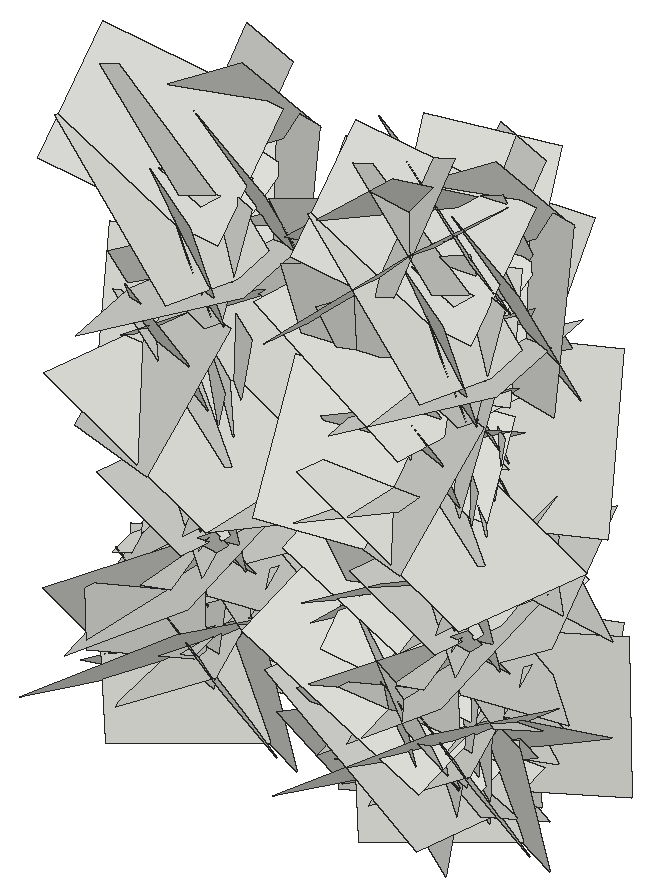
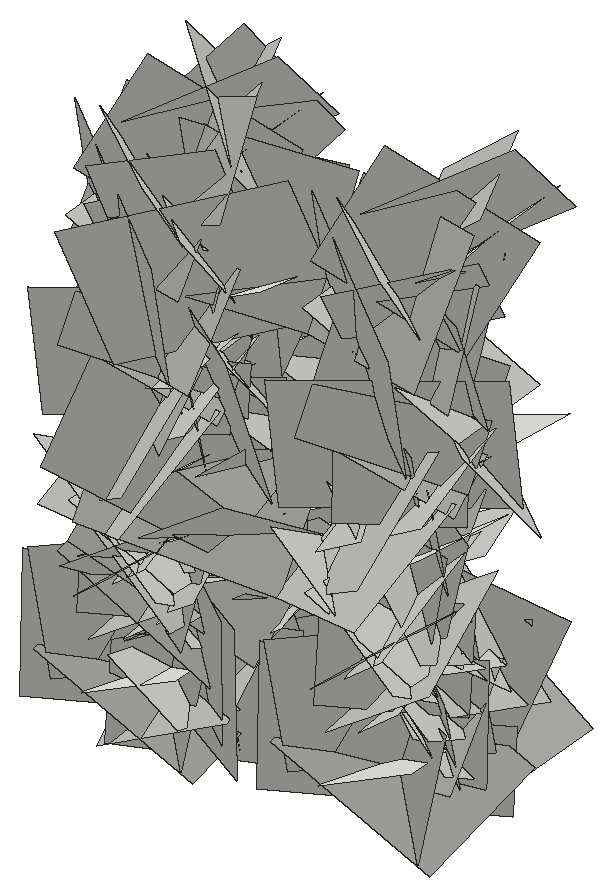
# SketchUp Ruby script. Lengths in inches.
U = 1.inch
M = Sketchup.active_model
def pt(a) = Geom::Point3d.new(a.map { |v| v * U })
def face(e, loops, mat)
  f = e.add_face(loops[0].map { |a| pt(a) })
  loops[1..].each { |l| e.add_face(l.map { |a| pt(a) }).erase! }
  f.material = f.back_material = mat if mat
  f
end
# faces: each face lists its corners as indices into pts; further lists are holes
def faces(e, pts, list, mat = nil) = list.each { |f| face(e, (f[0].is_a?(Array) ? f : [f]).map { |l| l.map { |i| pts[i] } }, mat) }
# xy, xz, yz: faces in a plane at the given z, y or x. An outline is a flat list of corners, or four numbers for a rectangle; further outlines are holes
def ring(l) = l.size == 4 ? [[l[0], l[1]], [l[2], l[1]], [l[2], l[3]], [l[0], l[3]]] : l.each_slice(2).to_a
def flat(e, list, mat, &to3) = list.each { |f| face(e, (f[0].is_a?(Array) ? f : [f]).map { |l| ring(l).map { |u, v| to3.(u, v) } }, mat) }
def xy(e, z, list, mat = nil) = flat(e, list, mat) { |x, y| [x, y, z] }
def xz(e, y, list, mat = nil) = flat(e, list, mat) { |x, z| [x, y, z] }
def yz(e, x, list, mat = nil) = flat(e, list, mat) { |y, z| [x, y, z] }
def lines(e, pts, list) = list.each { |a, b| e.add_line(pt(pts[a]), pt(pts[b])) }
# prism: a flat outline (further loops are holes) pulled along v
def prism(e, loops, v, mat = nil)
  f = face(e, loops, mat); d = Geom::Vector3d.new(v.map { |x| x * U })
  f.pushpull(f.normal.samedirection?(d) ? d.length : -d.length)
end
def box(e, o, s, mat = nil) = prism(e, [[o, [o[0] + s[0], o[1], o[2]], [o[0] + s[0], o[1] + s[1], o[2]], [o[0], o[1] + s[1], o[2]]]], [0, 0, s[2]], mat)
def at(x, y, z, deg = 0) = Geom::Transformation.translation(pt([x, y, z])) * Geom::Transformation.rotation(ORIGIN, Z_AXIS, deg.degrees)
def axes(o, x, y, z) = Geom::Transformation.new([*x, 0, *y, 0, *z, 0, *pt(o).to_a, 1])
def part(name) = M.definitions.add(name)
# library, detail: a bought-in or finely detailed component or shape, given as its bounding box
def library(name, o, s) = part(name).tap { |d| box(d.entities, o, s) }
def detail(e, o, s) = box(e.add_group.entities, o, s)
def put(e, d, t, mat = nil) = e.add_instance(d, t).tap { |i| i.material = mat if mat }
def group(e, t, mat = nil) = e.add_group.tap { |g| g.transformation = t; g.material = mat if mat }.entities
root = M.entities
c1 = part("Component\#6")
p = [[0.01,0,0],[0,3.24,4.54],[4.32,3.24,4.54],[4.33,0,0]]
faces(c1.entities,p,[[0,1,2,3]])
put(root,c1,axes([414.68,169.73,5.36],[-0.07377,0.11031,-0.61615],[-0.06228,-0.61836,-0.10407],[-0.66058,0.04598,0.07863]))
put(root,c1,axes([420.52,169.73,5.36],[0.07377,0.11031,-0.61615],[0.06228,-0.61836,-0.10407],[0.66058,0.04598,0.07863]))
put(root,c1,axes([424.49,169.73,5.36],[-0.07377,0.11031,-0.61615],[-0.06228,-0.61836,-0.10407],[-0.66058,0.04598,0.07863]))
put(root,c1,axes([414.68,170.45,6.95],[0.13562,-0.59571,0.16409],[-0.06684,0.15411,0.60864],[-0.65155,-0.13981,-0.02828]))
put(root,c1,axes([420.52,170.45,6.95],[-0.13562,-0.59571,0.16409],[0.06684,0.15411,0.60864],[0.65155,-0.13981,-0.02828]))
put(root,c1,axes([424.49,170.45,6.95],[0.13562,-0.59571,0.16409],[-0.06684,0.15411,0.60864],[-0.65155,-0.13981,-0.02828]))
put(root,c1,axes([410.71,172.51,13.7],[-0.18405,-0.71312,-0.93832],[-0.0125,-0.94735,0.72216],[1.2492,-0.11455,-0.13102]))
put(root,c1,axes([424.49,172.51,13.7],[0.18405,-0.71312,-0.93832],[0.0125,-0.94735,0.72216],[-1.2492,-0.11455,-0.13102]))
put(root,c1,axes([420.52,172.51,13.7],[-0.18405,-0.71312,-0.93832],[-0.0125,-0.94735,0.72216],[1.2492,-0.11455,-0.13102]))
put(root,c1,axes([410.71,166.89,12.83],[0.13197,1.26874,-0.04114],[0.28106,-0.06642,-1.24587],[1.31589,-0.11305,0.27023]))
put(root,c1,axes([424.49,166.89,12.83],[-0.13197,1.26874,-0.04114],[-0.28106,-0.06642,-1.24587],[-1.31589,-0.11305,0.27023]))
put(root,c1,axes([420.52,166.89,12.83],[0.13197,1.26874,-0.04114],[0.28106,-0.06642,-1.24587],[1.31589,-0.11305,0.27023]))
put(root,c1,axes([414.68,170.4375,18.81],[0.19883,-0.70321,0.38228],[0.06935,0.40479,0.71252],[-0.84558,-0.13215,0.14832]))
put(root,c1,axes([420.52,170.4375,18.81],[-0.19883,-0.70321,0.38228],[-0.06935,0.40479,0.71252],[0.84558,-0.13215,0.14832]))
put(root,c1,axes([424.49,170.4375,18.81],[0.19883,-0.70321,0.38228],[0.06935,0.40479,0.71252],[-0.84558,-0.13215,0.14832]))
put(root,c1,axes([410.71,172.01,0.23],[-0.18306,-1.21621,0.26629],[-0.00588,0.26959,1.22768],[1.31971,-0.16751,0.04241]))
put(root,c1,axes([424.49,172.01,0.23],[0.18306,-1.21621,0.26629],[0.00588,0.26959,1.22768],[-1.31971,-0.16751,0.04241]))
put(root,c1,axes([420.52,172.01,0.23],[-0.18306,-1.21621,0.26629],[-0.00588,0.26959,1.22768],[1.31971,-0.16751,0.04241]))
put(root,c1,axes([410.71,167.43,21.54],[0.05686,1.16606,-0.16138],[-0.18622,-0.15181,-1.15529],[1.23383,-0.07665,-0.16693]))
put(root,c1,axes([424.49,167.43,21.54],[-0.05686,1.16606,-0.16138],[0.18622,-0.15181,-1.15529],[-1.23383,-0.07665,-0.16693]))
put(root,c1,axes([420.52,167.43,21.54],[0.05686,1.16606,-0.16138],[-0.18622,-0.15181,-1.15529],[1.23383,-0.07665,-0.16693]))
put(root,c1,axes([410.71,170.29,20.28],[0.01759,0.35165,-0.94572],[0.09141,-0.94289,-0.34909],[1.06561,0.07508,0.04555]))
put(root,c1,axes([424.49,170.29,20.28],[-0.01759,0.35165,-0.94572],[-0.09141,-0.94289,-0.34909],[-1.06561,0.07508,0.04555]))
put(root,c1,axes([420.52,170.29,20.28],[0.01759,0.35165,-0.94572],[0.09141,-0.94289,-0.34909],[1.06561,0.07508,0.04555]))
put(root,c1,axes([410.71,166.61,20.4],[0.01588,0.7114,0.79833],[-0.18087,0.78977,-0.70057],[1.11894,0.11757,-0.12458]))
put(root,c1,axes([424.49,166.61,20.4],[-0.01588,0.7114,0.79833],[0.18087,0.78977,-0.70057],[-1.11894,0.11757,-0.12458]))
put(root,c1,axes([420.52,166.61,20.4],[0.01588,0.7114,0.79833],[-0.18087,0.78977,-0.70057],[1.11894,0.11757,-0.12458]))
put(root,c1,axes([414.68,169.875,11.58],[0.08121,-0.31714,0.54408],[-0.11401,0.53345,0.32609],[-0.65774,-0.13162,0.01065]))
put(root,c1,axes([420.52,169.875,11.58],[-0.08121,-0.31714,0.54408],[0.11401,0.53345,0.32609],[0.65774,-0.13162,0.01065]))
put(root,c1,axes([424.49,169.875,11.58],[0.08121,-0.31714,0.54408],[-0.11401,0.53345,0.32609],[-0.65774,-0.13162,0.01065]))
put(root,c1,axes([410.71,169.82,1.95],[-0.02915,-0.64251,0.76006],[-0.08177,0.75943,0.6392],[1.05178,0.04123,0.07076]))
put(root,c1,axes([424.49,169.82,1.95],[0.02915,-0.64251,0.76006],[0.08177,0.75943,0.6392],[-1.05178,0.04123,0.07076]))
put(root,c1,axes([420.52,169.82,1.95],[-0.02915,-0.64251,0.76006],[-0.08177,0.75943,0.6392],[1.05178,0.04123,0.07076]))
put(root,c1,axes([410.71,173.1,4.27],[0.006,-1.20261,-0.38975],[-0.07836,-0.3894,1.20046],[1.33775,-0.01742,0.07206]))
put(root,c1,axes([424.49,173.1,4.27],[-0.006,-1.20261,-0.38975],[0.07836,-0.3894,1.20046],[-1.33775,-0.01742,0.07206]))
put(root,c1,axes([420.52,173.1,4.27],[0.006,-1.20261,-0.38975],[-0.07836,-0.3894,1.20046],[1.33775,-0.01742,0.07206]))
put(root,c1,axes([414.68,169.57,7.53],[-0.02893,-0.34038,0.60393],[0.06424,0.60091,0.34142],[-0.73203,0.06619,0.00609]))
put(root,c1,axes([420.52,169.57,7.53],[0.02893,-0.34038,0.60393],[-0.06424,0.60091,0.34142],[0.73203,0.06619,0.00609]))
put(root,c1,axes([424.49,169.57,7.53],[-0.02893,-0.34038,0.60393],[0.06424,0.60091,0.34142],[-0.73203,0.06619,0.00609]))
put(root,c1,axes([410.71,172.68,14.25],[0.15371,-1.16437,-0.05617],[0.14183,-0.0396,1.1664],[1.22751,0.15038,-0.12774]))
put(root,c1,axes([424.49,172.68,14.25],[-0.15371,-1.16437,-0.05617],[-0.14183,-0.0396,1.1664],[-1.22751,0.15038,-0.12774]))
put(root,c1,axes([420.52,172.68,14.25],[0.15371,-1.16437,-0.05617],[0.14183,-0.0396,1.1664],[1.22751,0.15038,-0.12774]))
put(root,c1,axes([414.68,172.08,18.68],[0.05145,-0.65016,0.07549],[-0.09383,0.06848,0.64671],[-0.68743,-0.05801,-0.08262]))
put(root,c1,axes([424.49,172.08,18.68],[0.05145,-0.65016,0.07549],[-0.09383,0.06848,0.64671],[-0.68743,-0.05801,-0.08262]))
put(root,c1,axes([420.52,172.08,18.68],[-0.05145,-0.65016,0.07549],[0.09383,0.06848,0.64671],[0.68743,-0.05801,-0.08262]))
put(root,c1,axes([414.68,168.08,6.15],[0.10311,0.69666,0.5447],[0.01855,0.54636,-0.70191],[-0.9372,0.08746,0.04604]))
put(root,c1,axes([420.52,168.08,6.15],[-0.10311,0.69666,0.5447],[-0.01855,0.54636,-0.70191],[0.9372,0.08746,0.04604]))
put(root,c1,axes([424.49,168.08,6.15],[0.10311,0.69666,0.5447],[0.01855,0.54636,-0.70191],[-0.9372,0.08746,0.04604]))
put(root,c1,axes([410.71,170.37,5.28],[-0.04044,0.69271,-0.86885],[0.14808,-0.85947,-0.69137],[1.16852,0.13289,0.05755]))
put(root,c1,axes([424.49,170.37,5.28],[0.04044,0.69271,-0.86885],[-0.14808,-0.85947,-0.69137],[-1.16852,0.13289,0.05755]))
put(root,c1,axes([420.52,170.37,5.28],[-0.04044,0.69271,-0.86885],[0.14808,-0.85947,-0.69137],[1.16852,0.13289,0.05755]))
put(root,c1,axes([410.71,171.61,19.65],[-0.05512,0.44879,-0.89687],[-0.12411,-0.89465,-0.44089],[1.05579,-0.08174,-0.09865]))
put(root,c1,axes([424.49,171.61,19.65],[0.05512,0.44879,-0.89687],[0.12411,-0.89465,-0.44089],[-1.05579,-0.08174,-0.09865]))
put(root,c1,axes([420.52,171.61,19.65],[-0.05512,0.44879,-0.89687],[-0.12411,-0.89465,-0.44089],[1.05579,-0.08174,-0.09865]))
put(root,c1,axes([410.71,172.8125,18.6875],[-0.10377,-0.25363,-0.96814],[0.17625,-0.96337,0.23557],[1.04612,0.13715,-0.13572]))
put(root,c1,axes([424.49,172.8125,18.6875],[0.10377,-0.25363,-0.96814],[-0.17625,-0.96337,0.23557],[-1.04612,0.13715,-0.13572]))
put(root,c1,axes([420.52,172.8125,18.6875],[-0.10377,-0.25363,-0.96814],[0.17625,-0.96337,0.23557],[1.04612,0.13715,-0.13572]))
put(root,c1,axes([410.71,173.43,2.26],[0.13173,-0.86629,-0.47025],[-0.00519,-0.47451,0.87284],[1.04483,0.10686,0.06363]))
put(root,c1,axes([424.49,173.43,2.26],[-0.13173,-0.86629,-0.47025],[0.00519,-0.47451,0.87284],[-1.04483,0.10686,0.06363]))
put(root,c1,axes([420.52,173.43,2.26],[0.13173,-0.86629,-0.47025],[-0.00519,-0.47451,0.87284],[1.04483,0.10686,0.06363]))
put(root,c1,axes([414.68,172.62,2.82],[0.11022,-0.07985,-0.84847],[-0.01268,-0.85481,0.07898],[-0.90326,0.00226,-0.10464]))
put(root,c1,axes([420.52,172.62,2.82],[-0.11022,-0.07985,-0.84847],[0.01268,-0.85481,0.07898],[0.90326,0.00226,-0.10464]))
put(root,c1,axes([424.49,172.62,2.82],[0.11022,-0.07985,-0.84847],[-0.01268,-0.85481,0.07898],[-0.90326,0.00226,-0.10464]))
put(root,c1,axes([424.49,172.18,10.26],[-0.13568,0.14362,-0.9313],[-0.0793,-0.93844,-0.13444],[-0.9957,0.05517,0.13761]))
put(root,c1,axes([410.71,172.18,10.26],[0.13568,0.14362,-0.9313],[0.0793,-0.93844,-0.13444],[0.9957,0.05517,0.13761]))
put(root,c1,axes([420.52,172.18,10.26],[0.13568,0.14362,-0.9313],[0.0793,-0.93844,-0.13444],[0.9957,0.05517,0.13761]))
put(root,c1,axes([414.68,169.25,3.37],[0.12984,0.58451,0.34416],[0.01188,0.34794,-0.59491],[-0.71891,0.11132,0.05233]))
put(root,c1,axes([420.52,169.25,3.37],[-0.12984,0.58451,0.34416],[-0.01188,0.34794,-0.59491],[0.71891,0.11132,0.05233]))
put(root,c1,axes([424.49,169.25,3.37],[0.12984,0.58451,0.34416],[0.01188,0.34794,-0.59491],[-0.71891,0.11132,0.05233]))
put(root,c1,axes([410.71,174.625,6.88],[0.07025,-1.10898,-0.49527],[-0.16839,-0.49966,1.09755],[1.27636,-0.00489,0.17206]))
put(root,c1,axes([424.49,174.625,6.88],[-0.07025,-1.10898,-0.49527],[0.16839,-0.49966,1.09755],[-1.27636,-0.00489,0.17206]))
put(root,c1,axes([420.52,174.625,6.88],[0.07025,-1.10898,-0.49527],[-0.16839,-0.49966,1.09755],[1.27636,-0.00489,0.17206]))
put(root,c1,axes([410.71,173.47,4.9],[0.07332,-0.2848,-0.87141],[-0.0336,-0.87411,0.28317],[0.9712,-0.00874,0.07558]))
put(root,c1,axes([424.49,173.47,4.9],[-0.07332,-0.2848,-0.87141],[0.0336,-0.87411,0.28317],[-0.9712,-0.00874,0.07558]))
put(root,c1,axes([420.52,173.47,4.9],[0.07332,-0.2848,-0.87141],[-0.0336,-0.87411,0.28317],[0.9712,-0.00874,0.07558]))
put(root,c1,axes([414.68,169.67,8.54],[0.12628,0.08221,0.86907],[0.11161,0.86937,-0.09667],[-0.91857,0.11693,0.10773]))
put(root,c1,axes([420.52,169.67,8.54],[-0.12628,0.08221,0.86907],[-0.11161,0.86937,-0.09667],[0.91857,0.11693,0.10773]))
put(root,c1,axes([424.49,169.67,8.54],[0.12628,0.08221,0.86907],[0.11161,0.86937,-0.09667],[-0.91857,0.11693,0.10773]))
put(root,c1,axes([414.68,173.61,18.42],[-0.00387,-0.64214,-0.38262],[-0.01033,-0.38255,0.64212],[-0.79227,0.00812,-0.0065]))
put(root,c1,axes([420.52,173.61,18.42],[0.00387,-0.64214,-0.38262],[0.01033,-0.38255,0.64212],[0.79227,0.00812,-0.0065]))
put(root,c1,axes([424.49,173.61,18.42],[-0.00387,-0.64214,-0.38262],[-0.01033,-0.38255,0.64212],[-0.79227,0.00812,-0.0065]))
put(root,c1,axes([410.71,173.47,6.03],[-0.02519,-0.71274,-0.22366],[0.1783,-0.22314,0.69319],[0.7715,0.02829,-0.1675]))
put(root,c1,axes([424.49,173.47,6.03],[0.02519,-0.71274,-0.22366],[-0.1783,-0.22314,0.69319],[-0.7715,0.02829,-0.1675]))
put(root,c1,axes([420.52,173.47,6.03],[-0.02519,-0.71274,-0.22366],[0.1783,-0.22314,0.69319],[0.7715,0.02829,-0.1675]))
put(root,c1,axes([410.71,170.23,14.27],[-0.02775,1.05616,-0.50439],[-0.01222,-0.50473,-1.05626],[1.24058,0.01865,-0.02169]))
put(root,c1,axes([424.49,170.23,14.27],[0.02775,1.05616,-0.50439],[0.01222,-0.50473,-1.05626],[-1.24058,0.01865,-0.02169]))
put(root,c1,axes([420.52,170.23,14.27],[-0.02775,1.05616,-0.50439],[-0.01222,-0.50473,-1.05626],[1.24058,0.01865,-0.02169]))
put(root,c1,axes([410.71,172.3,17.31],[-0.17712,-0.66279,0.75583],[0.05377,0.75967,0.67737],[1.06423,-0.14869,0.09157]))
put(root,c1,axes([424.49,172.3,17.31],[0.17712,-0.66279,0.75583],[-0.05377,0.75967,0.67737],[-1.06423,-0.14869,0.09157]))
put(root,c1,axes([420.52,172.3,17.31],[-0.17712,-0.66279,0.75583],[0.05377,0.75967,0.67737],[1.06423,-0.14869,0.09157]))
put(root,c1,axes([410.71,171.9,21.66],[0.05821,0.63814,-1.10333],[0.23209,-1.09266,-0.62107],[1.33097,0.16262,0.15656]))
put(root,c1,axes([424.49,171.9,21.66],[-0.05821,0.63814,-1.10333],[-0.23209,-1.09266,-0.62107],[-1.33097,0.16262,0.15656]))
put(root,c1,axes([420.52,171.9,21.66],[0.05821,0.63814,-1.10333],[0.23209,-1.09266,-0.62107],[1.33097,0.16262,0.15656]))
put(root,c1,axes([414.68,171.64,6.09],[0.04085,-0.22846,0.61977],[-0.06336,0.61707,0.23119],[-0.6973,-0.06945,0.0153]))
put(root,c1,axes([420.52,171.64,6.09],[-0.04085,-0.22846,0.61977],[0.06336,0.61707,0.23119],[0.6973,-0.06945,0.0153]))
put(root,c1,axes([424.49,171.64,6.09],[0.04085,-0.22846,0.61977],[-0.06336,0.61707,0.23119],[-0.6973,-0.06945,0.0153]))
put(root,c1,axes([410.71,170.14,10.52],[0.06349,0.95893,0.01002],[-0.03302,0.01198,-0.96028],[1.01599,-0.05954,-0.03183]))
put(root,c1,axes([424.49,170.14,10.52],[-0.06349,0.95893,0.01002],[0.03302,0.01198,-0.96028],[-1.01599,-0.05954,-0.03183]))
put(root,c1,axes([420.52,170.14,10.52],[0.06349,0.95893,0.01002],[-0.03302,0.01198,-0.96028],[1.01599,-0.05954,-0.03183]))
put(root,c1,axes([414.68,174.87,19.3],[0.1513,-0.51657,-0.73784],[0.06675,-0.7395,0.52991],[-0.9524,-0.13389,-0.08008]))
put(root,c1,axes([420.52,174.87,19.3],[-0.1513,-0.51657,-0.73784],[-0.06675,-0.7395,0.52991],[0.9524,-0.13389,-0.08008]))
put(root,c1,axes([424.49,174.87,19.3],[0.1513,-0.51657,-0.73784],[0.06675,-0.7395,0.52991],[-0.9524,-0.13389,-0.08008]))
put(root,c1,axes([410.71,172.92,11.6],[0.15777,-0.72106,0.34948],[-0.01112,0.35368,0.73418],[0.84929,0.13857,-0.05531]))
put(root,c1,axes([424.49,172.92,11.6],[-0.15777,-0.72106,0.34948],[0.01112,0.35368,0.73418],[-0.84929,0.13857,-0.05531]))
put(root,c1,axes([420.52,172.92,11.6],[0.15777,-0.72106,0.34948],[-0.01112,0.35368,0.73418],[0.84929,0.13857,-0.05531]))
put(root,c1,axes([410.71,169.35,10.4],[-0.15861,0.37048,1.309],[0.06067,1.31744,-0.36632],[1.44077,-0.01469,0.15953]))
put(root,c1,axes([424.49,169.35,10.4],[0.15861,0.37048,1.309],[-0.06067,1.31744,-0.36632],[-1.44077,-0.01469,0.15953]))
put(root,c1,axes([420.52,169.35,10.4],[-0.15861,0.37048,1.309],[0.06067,1.31744,-0.36632],[1.44077,-0.01469,0.15953]))
put(root,c1,axes([410.71,171.5,10.51],[0.09816,1.08592,-0.68794],[-0.27584,-0.65961,-1.07622],[1.33441,-0.21623,-0.17187]))
put(root,c1,axes([424.49,171.5,10.51],[-0.09816,1.08592,-0.68794],[0.27584,-0.65961,-1.07622],[-1.33441,-0.21623,-0.17187]))
put(root,c1,axes([420.52,171.5,10.51],[0.09816,1.08592,-0.68794],[-0.27584,-0.65961,-1.07622],[1.33441,-0.21623,-0.17187]))
put(root,c1,axes([410.71,170.67,8.7],[-0.18467,1.04701,-0.56036],[-0.0341,-0.57031,-1.0556],[1.25832,0.1382,-0.11085]))
put(root,c1,axes([424.49,170.67,8.7],[0.18467,1.04701,-0.56036],[0.0341,-0.57031,-1.0556],[-1.25832,0.1382,-0.11085]))
put(root,c1,axes([420.52,170.67,8.7],[-0.18467,1.04701,-0.56036],[-0.0341,-0.57031,-1.0556],[1.25832,0.1382,-0.11085]))
put(root,c1,axes([410.71,174.22,3.89],[0.08779,-0.72671,-0.31501],[0.02258,-0.31457,0.73129],[0.83927,0.08448,0.01327]))
put(root,c1,axes([424.49,174.22,3.89],[-0.08779,-0.72671,-0.31501],[-0.02258,-0.31457,0.73129],[-0.83927,0.08448,0.01327]))
put(root,c1,axes([420.52,174.22,3.89],[0.08779,-0.72671,-0.31501],[0.02258,-0.31457,0.73129],[0.83927,0.08448,0.01327]))
put(root,c1,axes([410.71,174.19,-1.125],[-0.19779,-1.01545,0.55728],[0.13113,0.54376,1.03224],[1.22079,-0.22293,-0.02059]))
put(root,c1,axes([424.49,174.19,-1.125],[0.19779,-1.01545,0.55728],[-0.13113,0.54376,1.03224],[-1.22079,-0.22293,-0.02059]))
put(root,c1,axes([420.52,174.19,-1.125],[-0.19779,-1.01545,0.55728],[0.13113,0.54376,1.03224],[1.22079,-0.22293,-0.02059]))
put(root,c1,axes([414.68,171.41,10.85],[0.07762,0.04197,0.59758],[-0.0194,0.6019,-0.04003],[-0.6347,-0.01326,0.07431]))
put(root,c1,axes([420.52,171.41,10.85],[-0.07762,0.04197,0.59758],[0.0194,0.6019,-0.04003],[0.6347,-0.01326,0.07431]))
put(root,c1,axes([424.49,171.41,10.85],[0.07762,0.04197,0.59758],[-0.0194,0.6019,-0.04003],[-0.6347,-0.01326,0.07431]))
put(root,c1,axes([410.71,173.32,3.72],[0.0912,0.22313,-1.04907],[0.17676,-1.04242,-0.20804],[1.12306,0.14594,0.11794]))
put(root,c1,axes([424.49,173.32,3.72],[-0.0912,0.22313,-1.04907],[-0.17676,-1.04242,-0.20804],[-1.12306,0.14594,0.11794]))
put(root,c1,axes([420.52,173.32,3.72],[0.0912,0.22313,-1.04907],[0.17676,-1.04242,-0.20804],[1.12306,0.14594,0.11794]))
put(root,c1,axes([414.68,173.27,2.31],[-0.02745,-0.60704,0.2793],[0.09658,0.2737,0.6033],[-0.70169,0.06142,0.07211]))
put(root,c1,axes([420.52,173.27,2.31],[0.02745,-0.60704,0.2793],[-0.09658,0.2737,0.6033],[0.70169,0.06142,0.07211]))
put(root,c1,axes([424.49,173.27,2.31],[-0.02745,-0.60704,0.2793],[0.09658,0.2737,0.6033],[-0.70169,0.06142,0.07211]))
put(root,c1,axes([410.71,172.23,12.17],[0.04321,-0.56467,0.8488],[-0.06772,0.84639,0.56613],[1.07851,0.07577,0.00154]))
put(root,c1,axes([424.49,172.23,12.17],[-0.04321,-0.56467,0.8488],[0.06772,0.84639,0.56613],[-1.07851,0.07577,0.00154]))
put(root,c1,axes([420.52,172.23,12.17],[0.04321,-0.56467,0.8488],[-0.06772,0.84639,0.56613],[1.07851,0.07577,0.00154]))
put(root,c1,axes([410.71,170.77,1.94],[0.10305,0.14958,1.1623],[-0.03,1.16625,-0.14772],[1.24184,0.01576,-0.10002]))
put(root,c1,axes([424.49,170.77,1.94],[-0.10305,0.14958,1.1623],[0.03,1.16625,-0.14772],[-1.24184,0.01576,-0.10002]))
put(root,c1,axes([420.52,170.77,1.94],[0.10305,0.14958,1.1623],[-0.03,1.16625,-0.14772],[1.24184,0.01576,-0.10002]))
put(root,c1,axes([410.71,172.28,10.96],[0.19399,-0.26613,0.68464],[-0.06344,0.69782,0.28725],[0.77602,0.12358,-0.14766]))
put(root,c1,axes([424.49,172.28,10.96],[-0.19399,-0.26613,0.68464],[0.06344,0.69782,0.28725],[-0.77602,0.12358,-0.14766]))
put(root,c1,axes([420.52,172.28,10.96],[0.19399,-0.26613,0.68464],[-0.06344,0.69782,0.28725],[0.77602,0.12358,-0.14766]))
put(root,c1,axes([410.71,172.17,3.88],[0.10658,-0.21665,0.83392],[-0.00523,0.83942,0.21867],[0.91328,0.03009,-0.09606]))
put(root,c1,axes([424.49,172.17,3.88],[-0.10658,-0.21665,0.83392],[0.00523,0.83942,0.21867],[-0.91328,0.03009,-0.09606]))
put(root,c1,axes([420.52,172.17,3.88],[0.10658,-0.21665,0.83392],[-0.00523,0.83942,0.21867],[0.91328,0.03009,-0.09606]))
put(root,c1,axes([410.71,172.79,12.08],[0.24348,0.91998,-0.78066],[0.03668,-0.79938,-0.93185],[1.27843,-0.15228,0.17542]))
put(root,c1,axes([424.49,172.79,12.08],[-0.24348,0.91998,-0.78066],[-0.03668,-0.79938,-0.93185],[-1.27843,-0.15228,0.17542]))
put(root,c1,axes([420.52,172.79,12.08],[0.24348,0.91998,-0.78066],[0.03668,-0.79938,-0.93185],[1.27843,-0.15228,0.17542]))
put(root,c1,axes([424.49,171.28,0.09],[0.0277,-0.00252,1.28462],[-0.09278,1.2819,0.0043],[-1.35854,-0.08759,0.0259]))
put(root,c1,axes([410.71,171.28,0.09],[-0.0277,-0.00252,1.28462],[0.09278,1.2819,0.0043],[1.35854,-0.08759,0.0259]))
put(root,c1,axes([420.52,171.28,0.09],[-0.0277,-0.00252,1.28462],[0.09278,1.2819,0.0043],[1.35854,-0.08759,0.0259]))
put(root,c1,axes([414.68,174.97,1.18],[0.10067,-0.62121,-0.06126],[-0.13552,-0.08001,0.61313],[-0.64765,-0.07982,-0.13782]))
put(root,c1,axes([420.52,174.97,1.18],[-0.10067,-0.62121,-0.06126],[0.13552,-0.08001,0.61313],[0.64765,-0.07982,-0.13782]))
put(root,c1,axes([424.49,174.97,1.18],[0.10067,-0.62121,-0.06126],[-0.13552,-0.08001,0.61313],[-0.64765,-0.07982,-0.13782]))
put(root,c1,axes([410.71,176.36,18.92],[0.19548,-0.4632,-1.27504],[-0.04093,-1.28804,0.46234],[1.43738,0.02631,0.18657]))
put(root,c1,axes([424.49,176.36,18.92],[-0.19548,-0.4632,-1.27504],[0.04093,-1.28804,0.46234],[-1.43738,0.02631,0.18657]))
put(root,c1,axes([420.52,176.36,18.92],[0.19548,-0.4632,-1.27504],[-0.04093,-1.28804,0.46234],[1.43738,0.02631,0.18657]))
put(root,c1,axes([410.71,176.11,6.43],[0.23133,-1.0261,-0.61864],[0.04368,-0.62202,1.04624],[1.2693,0.20842,0.07674]))
put(root,c1,axes([424.49,176.11,6.43],[-0.23133,-1.0261,-0.61864],[-0.04368,-0.62202,1.04624],[-1.2693,0.20842,0.07674]))
put(root,c1,axes([420.52,176.11,6.43],[0.23133,-1.0261,-0.61864],[0.04368,-0.62202,1.04624],[1.2693,0.20842,0.07674]))
put(root,c1,axes([410.71,175.17,6.35],[0.11089,-0.78923,-0.08985],[0.10937,-0.07636,0.79084],[0.83485,0.11483,-0.09167]))
put(root,c1,axes([424.49,175.17,6.35],[-0.11089,-0.78923,-0.08985],[-0.10937,-0.07636,0.79084],[-0.83485,0.11483,-0.09167]))
put(root,c1,axes([420.52,175.17,6.35],[0.11089,-0.78923,-0.08985],[0.10937,-0.07636,0.79084],[0.83485,0.11483,-0.09167]))
put(root,c1,axes([414.68,175.4,4.97],[-0.01432,-0.74639,-0.04739],[0.08616,-0.04858,0.74199],[-0.78807,0.00825,0.08199]))
put(root,c1,axes([420.52,175.4,4.97],[0.01432,-0.74639,-0.04739],[-0.08616,-0.04858,0.74199],[0.78807,0.00825,0.08199]))
put(root,c1,axes([424.49,175.4,4.97],[-0.01432,-0.74639,-0.04739],[0.08616,-0.04858,0.74199],[-0.78807,0.00825,0.08199]))
put(root,c1,axes([410.71,173.68,14.42],[0.07839,0.88361,-0.83437],[-0.27617,-0.80495,-0.87555],[1.25826,-0.23172,-0.14019]))
put(root,c1,axes([424.49,173.68,14.42],[-0.07839,0.88361,-0.83437],[0.27617,-0.80495,-0.87555],[-1.25826,-0.23172,-0.14019]))
put(root,c1,axes([420.52,173.68,14.42],[0.07839,0.88361,-0.83437],[-0.27617,-0.80495,-0.87555],[1.25826,-0.23172,-0.14019]))
put(root,c1,axes([414.68,171.94,19.49],[0.08782,0.36838,0.63269],[-0.00702,0.63708,-0.37006],[-0.77601,0.03592,0.07495]))
put(root,c1,axes([420.52,171.94,19.49],[-0.08782,0.36838,0.63269],[0.00702,0.63708,-0.37006],[0.77601,0.03592,0.07495]))
put(root,c1,axes([424.49,171.94,19.49],[0.08782,0.36838,0.63269],[-0.00702,0.63708,-0.37006],[-0.77601,0.03592,0.07495]))
